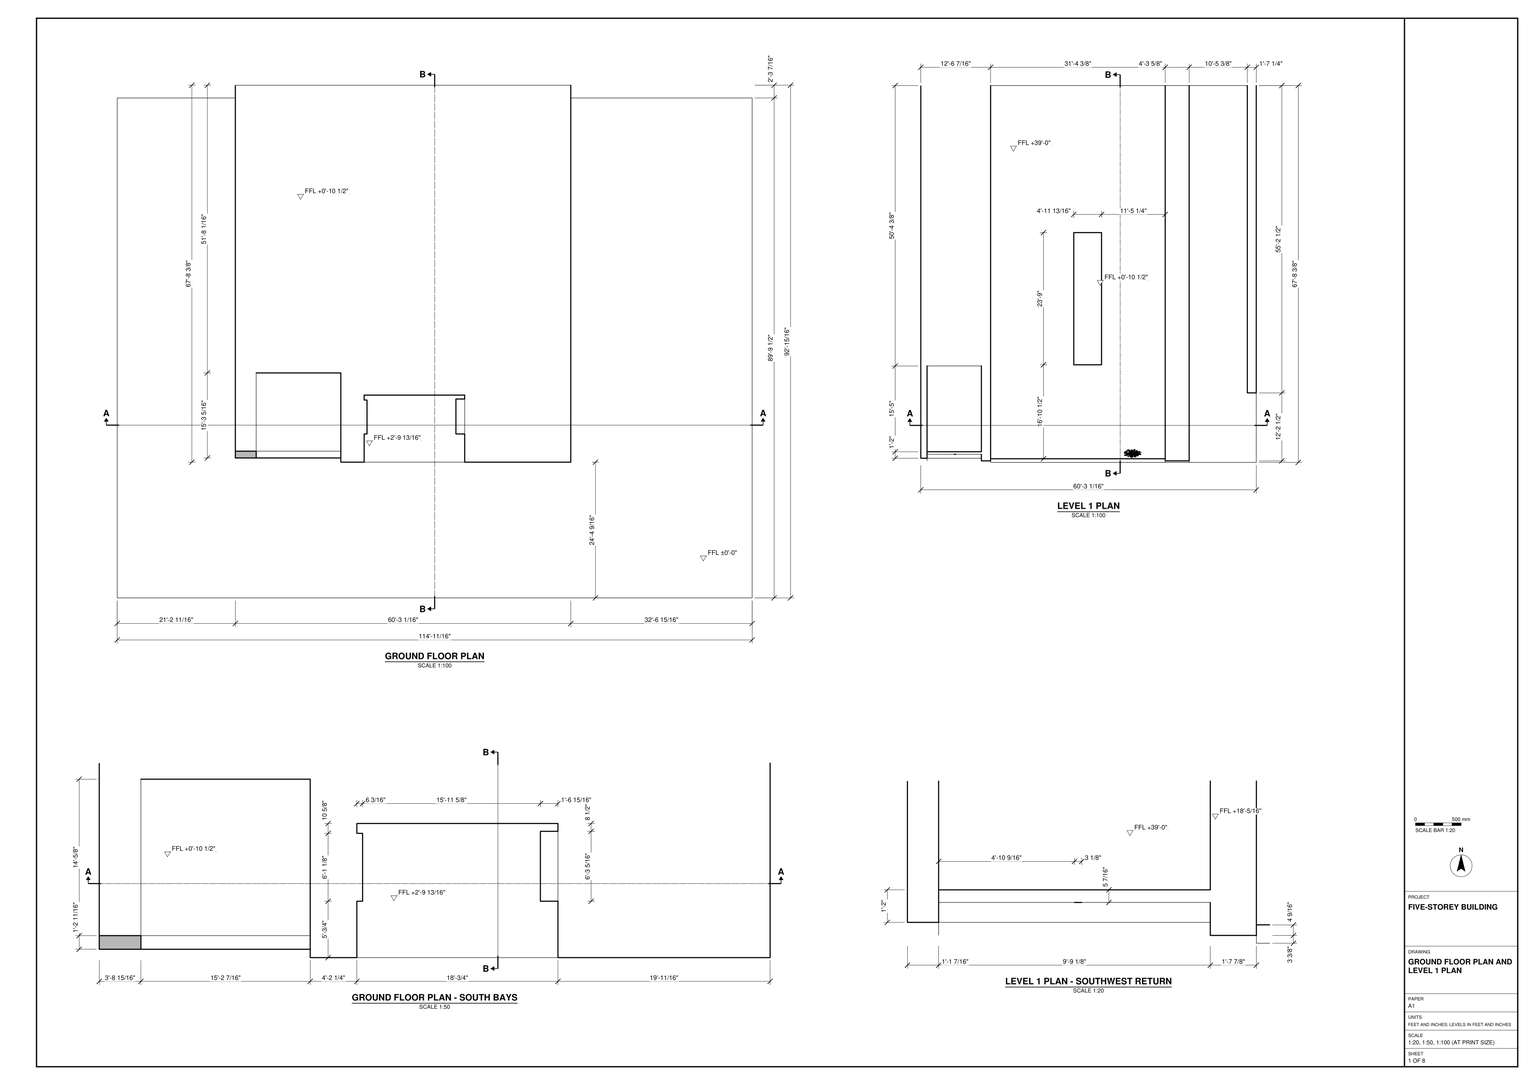
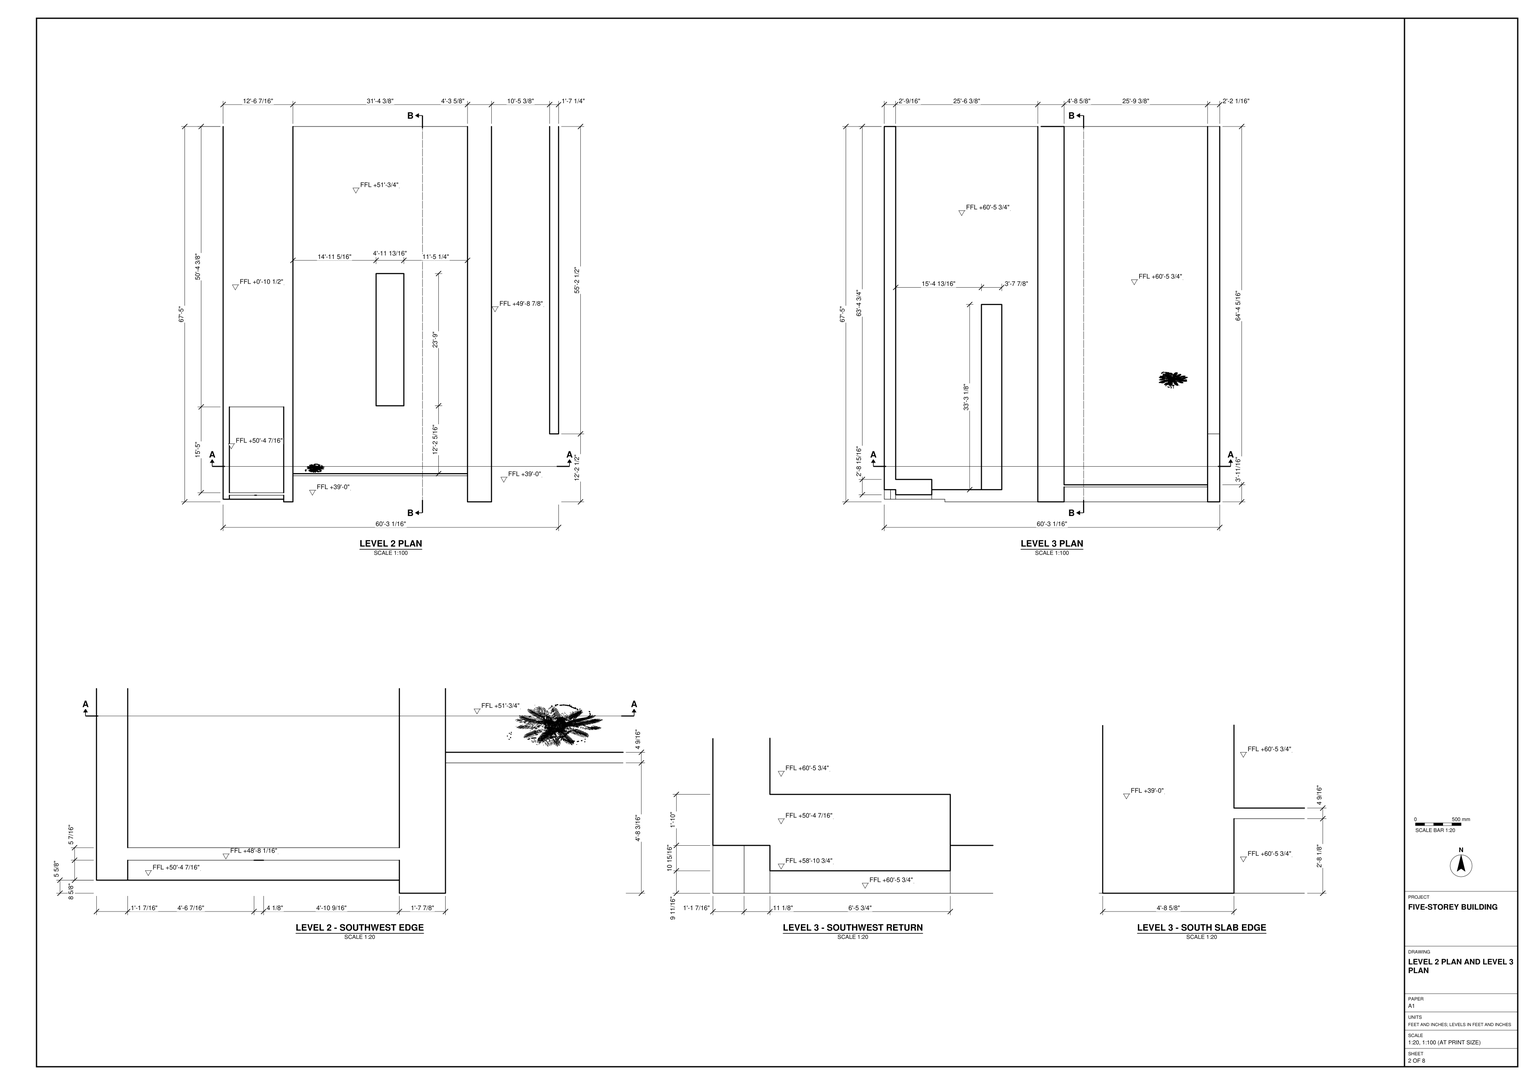
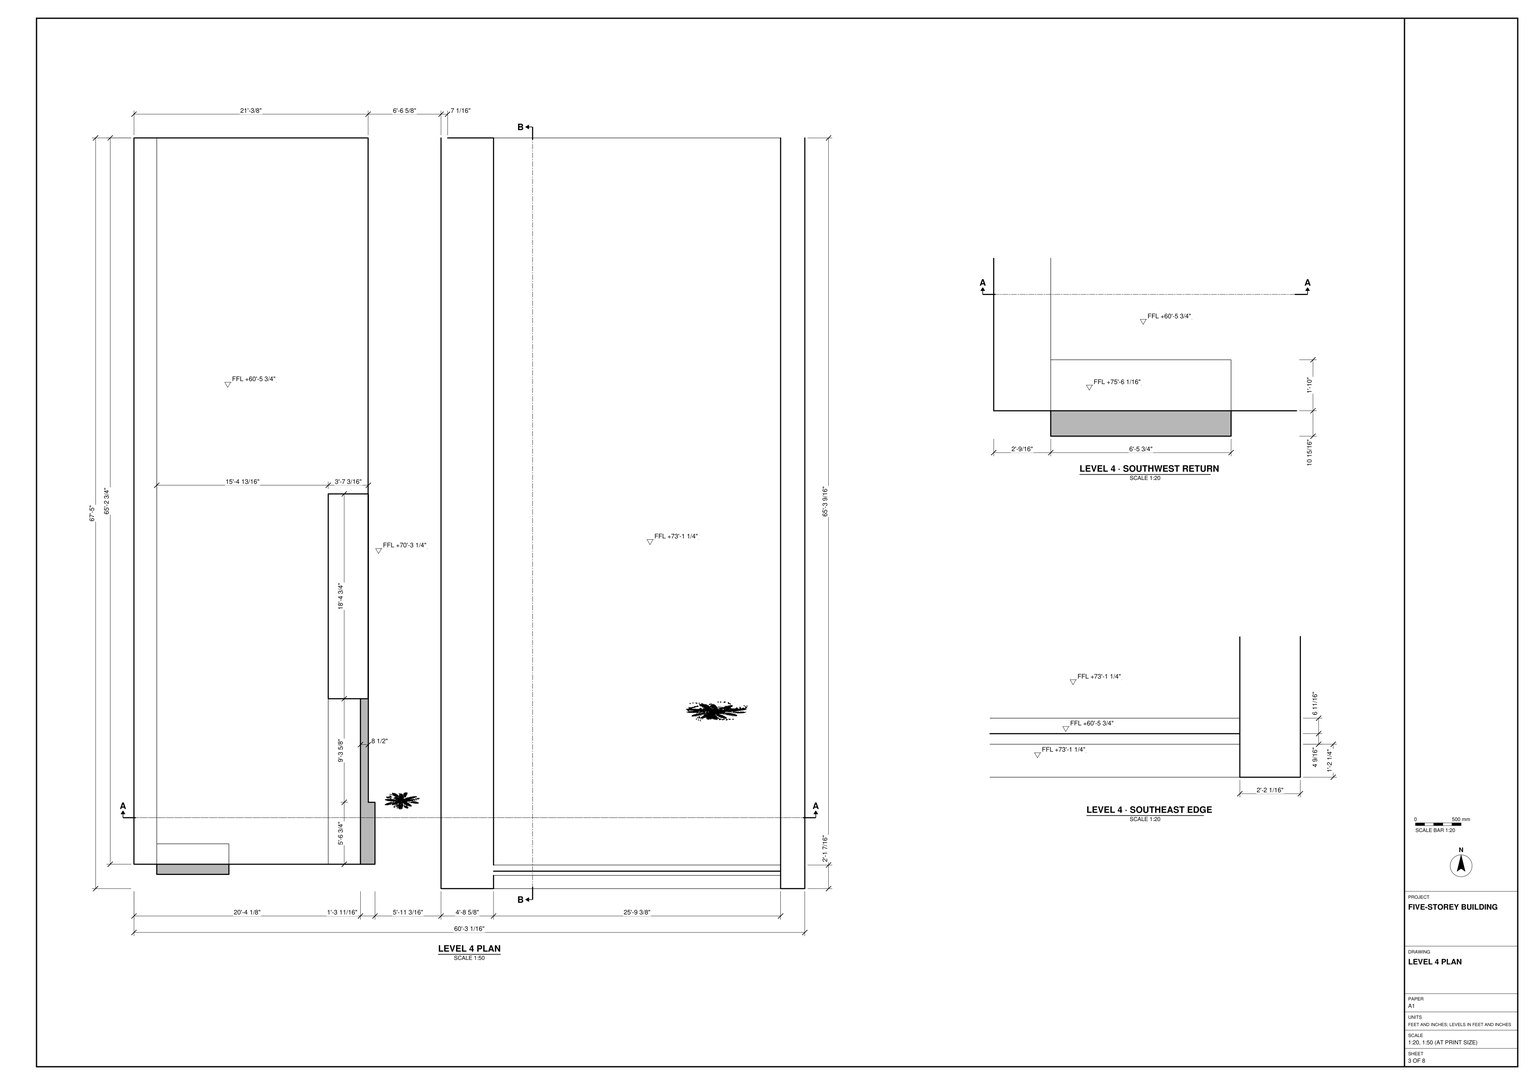
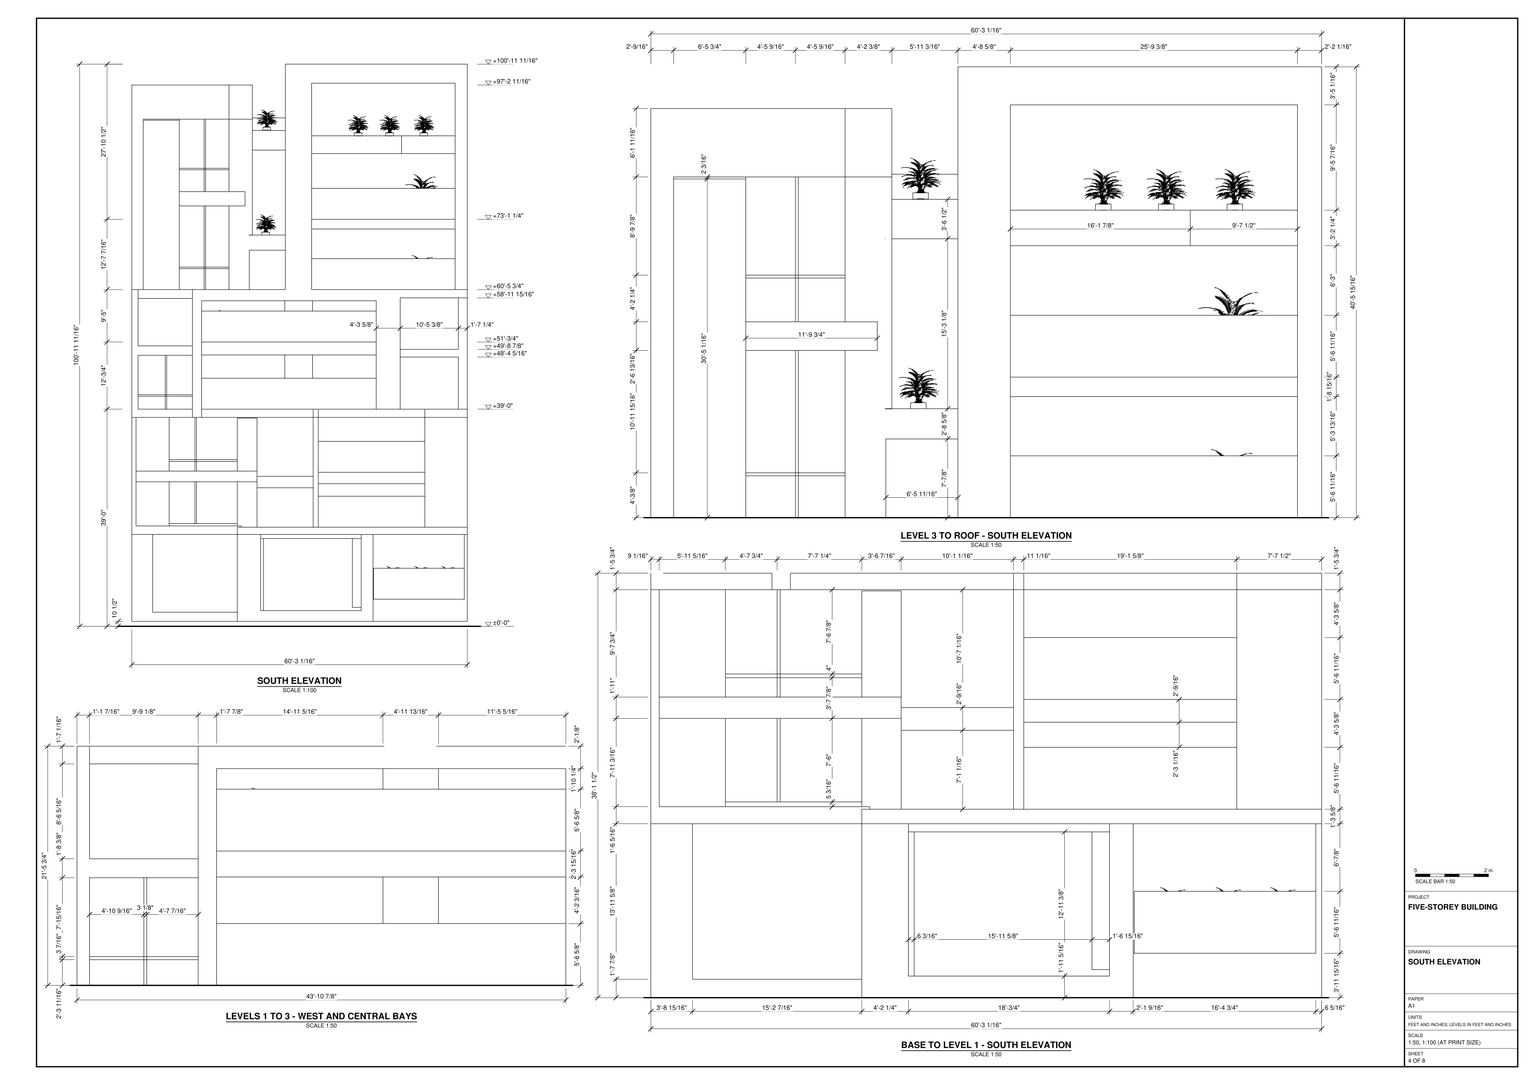
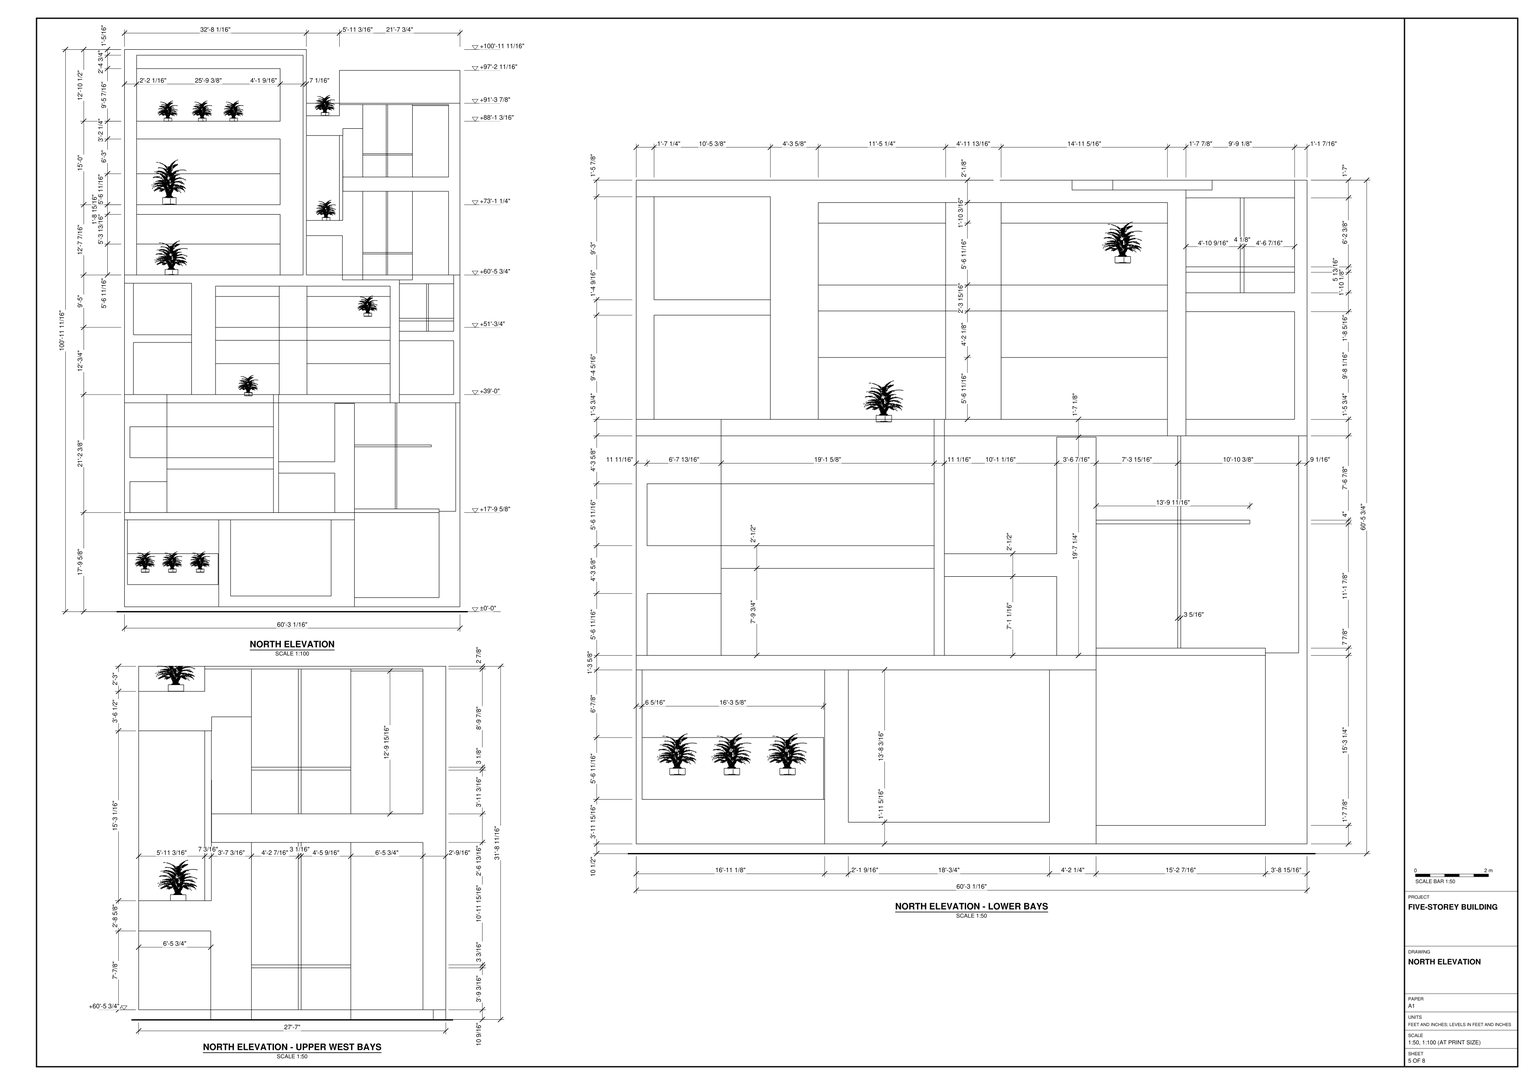
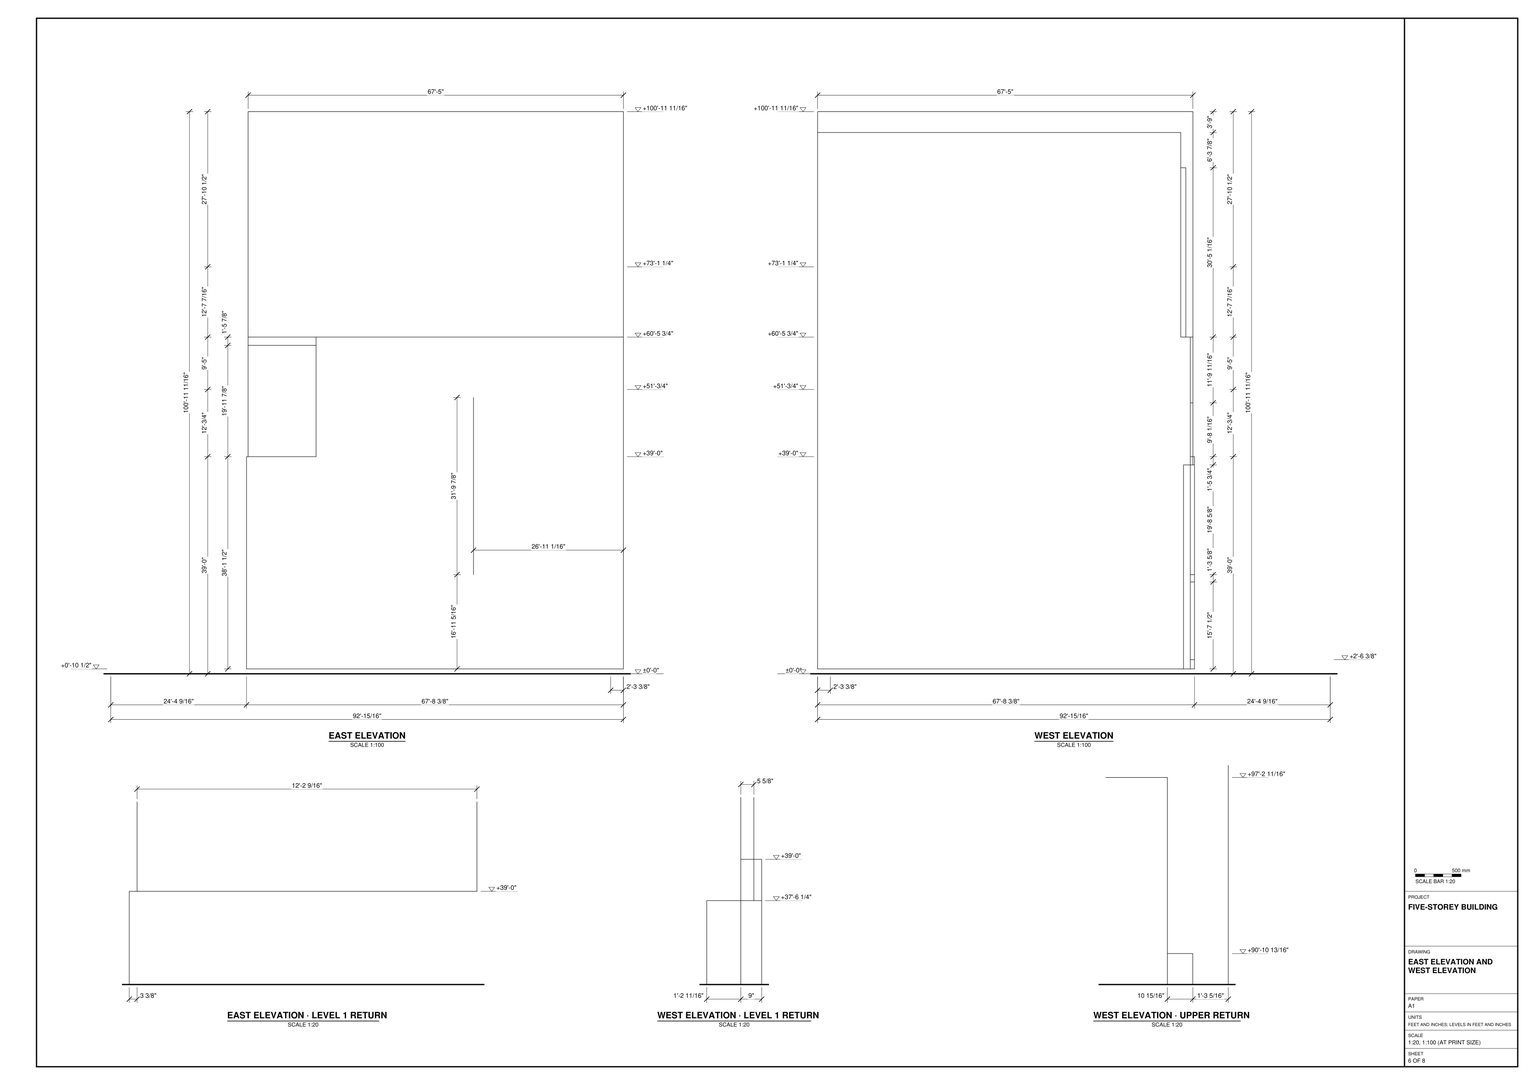
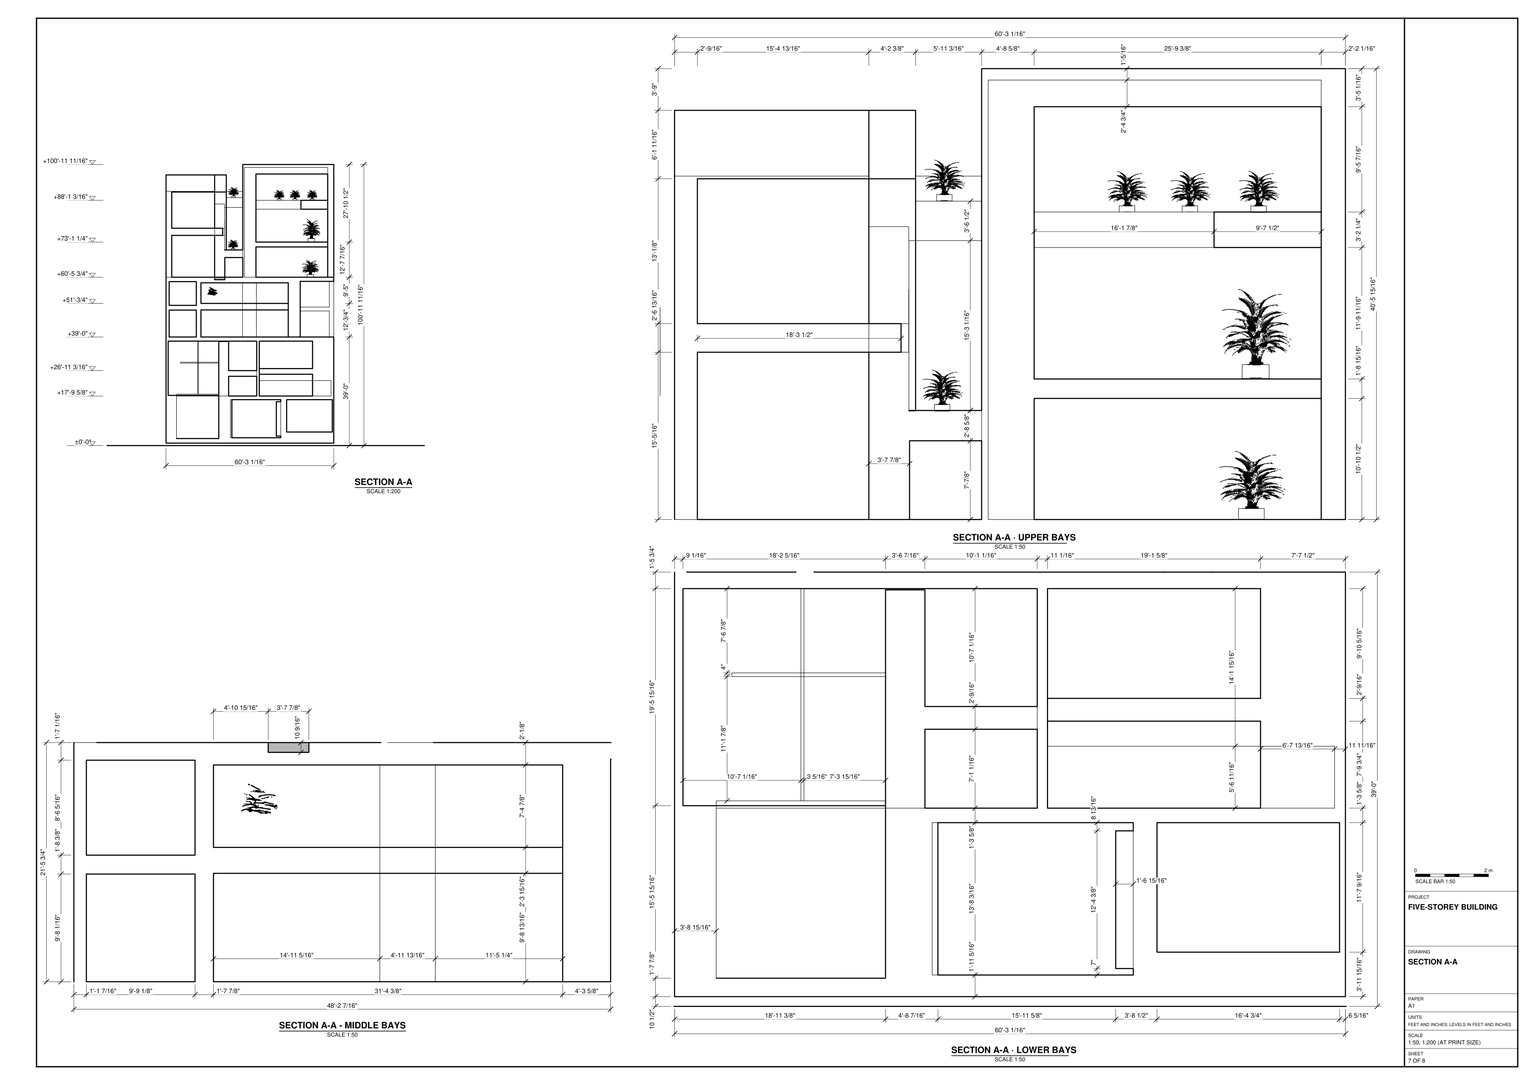
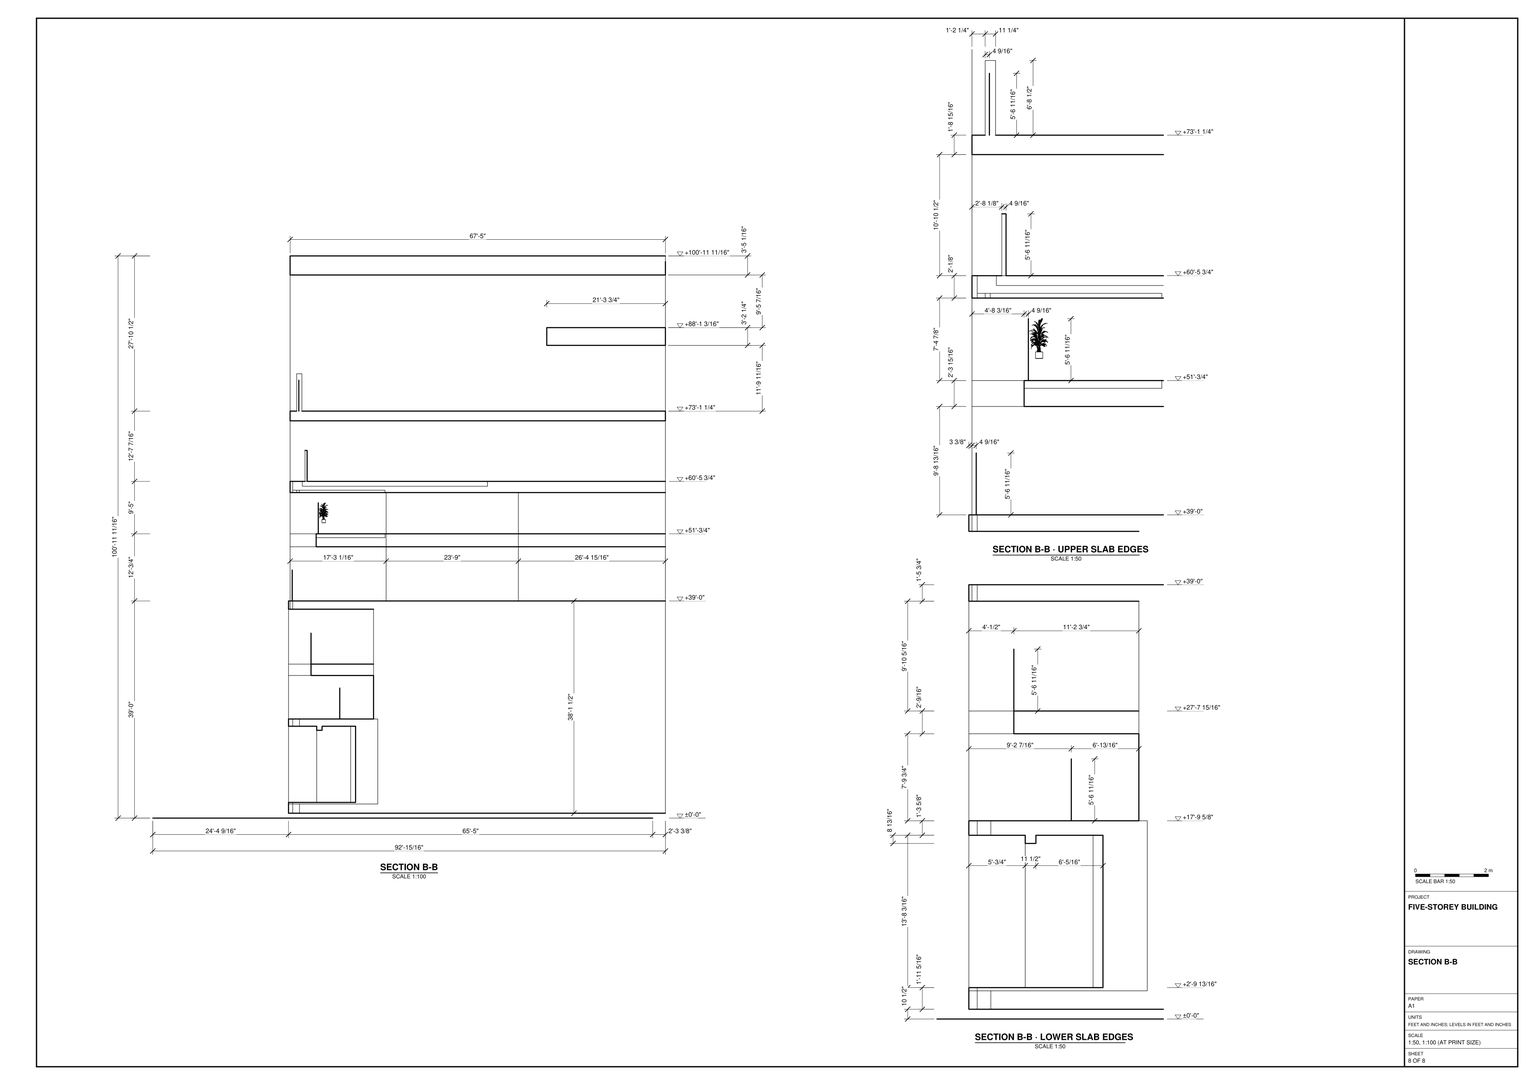
Build the five-storey building in SketchUp from task_files/diagram_01.pdf. Work in feet and inches. Including the site, the model shall span 114'-11/16" along X, 92'-15/16" along Y and 100'-11 11/16" along Z. Set the ground datum at ±0'-0" and the successive principal levels at +39'-0", +51'-3/4", +60'-5 3/4" and +73'-1 1/4".

Use the ground-floor plan to place the building on the site, leaving the open area to the south and the unequal margins to the west and east. Shape the south bays from the enlarged plan. Build each upper slab from its own outline rather than copying the ground footprint upwards. Preserve the long opening in the lower slabs, the stepped southwest returns and the change in height between the east and west portions at the top. Follow the sheets for wall thicknesses, openings, slab edges and roof profiles; include stairs, built-in joinery and main furniture where shown.

Keep walls, slabs and roof elements in separate groups or components, group each furniture or joinery piece separately, and use components for repeated parts. Plants and other loose or decorative items may be any suitable library components. Save one SketchUp model as output_files/five_storey_building_and_its_site.skp.

# SketchUp Ruby script. Lengths in inches.
U = 1.inch
M = Sketchup.active_model
def pt(a) = Geom::Point3d.new(a.map { |v| v * U })
def face(e, loops, mat)
  f = e.add_face(loops[0].map { |a| pt(a) })
  loops[1..].each { |l| e.add_face(l.map { |a| pt(a) }).erase! }
  f.material = f.back_material = mat if mat
  f
end
# faces: each face lists its corners as indices into pts; further lists are holes
def faces(e, pts, list, mat = nil) = list.each { |f| face(e, (f[0].is_a?(Array) ? f : [f]).map { |l| l.map { |i| pts[i] } }, mat) }
# xy, xz, yz: faces in a plane at the given z, y or x. An outline is a flat list of corners, or four numbers for a rectangle; further outlines are holes
def ring(l) = l.size == 4 ? [[l[0], l[1]], [l[2], l[1]], [l[2], l[3]], [l[0], l[3]]] : l.each_slice(2).to_a
def flat(e, list, mat, &to3) = list.each { |f| face(e, (f[0].is_a?(Array) ? f : [f]).map { |l| ring(l).map { |u, v| to3.(u, v) } }, mat) }
def xy(e, z, list, mat = nil) = flat(e, list, mat) { |x, y| [x, y, z] }
def xz(e, y, list, mat = nil) = flat(e, list, mat) { |x, z| [x, y, z] }
def yz(e, x, list, mat = nil) = flat(e, list, mat) { |y, z| [x, y, z] }
def lines(e, pts, list) = list.each { |a, b| e.add_line(pt(pts[a]), pt(pts[b])) }
# prism: a flat outline (further loops are holes) pulled along v
def prism(e, loops, v, mat = nil)
  f = face(e, loops, mat); d = Geom::Vector3d.new(v.map { |x| x * U })
  f.pushpull(f.normal.samedirection?(d) ? d.length : -d.length)
end
def box(e, o, s, mat = nil) = prism(e, [[o, [o[0] + s[0], o[1], o[2]], [o[0] + s[0], o[1] + s[1], o[2]], [o[0], o[1] + s[1], o[2]]]], [0, 0, s[2]], mat)
def at(x, y, z, deg = 0) = Geom::Transformation.translation(pt([x, y, z])) * Geom::Transformation.rotation(ORIGIN, Z_AXIS, deg.degrees)
def axes(o, x, y, z) = Geom::Transformation.new([*x, 0, *y, 0, *z, 0, *pt(o).to_a, 1])
def part(name) = M.definitions.add(name)
# library, detail: a bought-in or finely detailed component or shape, given as its bounding box
def library(name, o, s) = part(name).tap { |d| box(d.entities, o, s) }
def detail(e, o, s) = box(e.add_group.entities, o, s)
def put(e, d, t, mat = nil) = e.add_instance(d, t).tap { |i| i.material = mat if mat }
def group(e, t, mat = nil) = e.add_group.tap { |g| g.transformation = t; g.material = mat if mat }.entities
root = M.entities
M.materials.add("Niraj_Hair_Gray").color = [178, 178, 178]
M.materials.add("[Asphalt New]").color = [67, 60, 62]
M.materials.add("[Translucent Glass Gray]").color = [128, 128, 128]
M.materials["[Translucent Glass Gray]"].alpha = 0.5
c1 = library("plant_176_fbx.FBX\#1",[-22.43,-22.29,0],[44.86,44.58,89.56])
c2 = part("plant")
put(c2.entities,c1,axes([-237.41,482.42,160.98],[1.055,0,0],[0,0.5,0],[0,0,0.5]))
put(c2.entities,c1,axes([-237.41,591.17,160.98],[1.055,0,0],[0,0.5,0],[0,0,0.5]))
put(c2.entities,c1,axes([-237.41,699.92,160.98],[1.055,0,0],[0,0.5,0],[0,0,0.5]))
put(c2.entities,c1,axes([-237.41,808.67,160.98],[1.055,0,0],[0,0.5,0],[0,0,0.5]))
put(c2.entities,c1,axes([-237.41,917.42,160.98],[1.055,0,0],[0,0.5,0],[0,0,0.5]))
put(c2.entities,c1,axes([-237.41,1026.17,160.98],[1.055,0,0],[0,0.5,0],[0,0,0.5]))
put(c2.entities,c1,axes([-311.35,1134.92,160.98],[1.055,0,0],[0,0.5,0],[0,0,0.5]))
put(c2.entities,c1,axes([-379.16,1134.92,160.98],[1.055,0,0],[0,0.5,0],[0,0,0.5]))
put(c2.entities,c1,axes([-240.46,645.63,-18.48],[1.8357,0,0],[0,0.5,0],[0,0,1.09]))
put(c2.entities,c1,axes([-245.08,718.66,-169.93],[1.7513,0,0],[0,0.83,0],[0,0,0.83]))
put(c2.entities,c1,axes([-576.07,586.95,173.15],[1.055,0,0],[0,0.5,0],[0,0,0.5]))
put(c2.entities,c1,axes([-578.43,549.41,-53.08],[1.055,0,0],[0,0.5,0],[0,0,0.5]))
put(c2.entities,c1,axes([-410.75,470.8,-430.43],[1.055,0,0],[0,0.5,0],[0,0,0.5]))
put(c2.entities,c1,axes([-668.22,526.99,-259.24],[1.055,0,0],[0,0.5,0],[0,0,0.5]))
put(c2.entities,c1,axes([-246.96,495.71,-810.87],[1.055,0,0],[0,0.5,0],[0,0,0.5]))
put(c2.entities,c1,axes([-188.27,495.71,-810.87],[1.055,0,0],[0,0.5,0],[0,0,0.5]))
put(c2.entities,c1,axes([-306.89,495.71,-810.87],[1.055,0,0],[0,0.5,0],[0,0,0.5]))
xy(root,-10.52,[[0,0,1368.6875,1077.5]])
xy(root,0,[[482.05,292.54,977.74,292.54,977.74,1104.91,254.67,1104.91,254.67,316.23,482.05,316.23],[254.67,301.54,482.05,316.23]])
xy(root,19.86,[[299.59,301.54,482.05,316.23],[299.59,316.23,482.05,484.85]])
xy(root,23.3,[[532.33,292.54,749.08,292.54,749.08,437.1,532.33,437.1,532.33,426.45,538.51,426.45,538.51,353.31,532.33,353.31]])
xy(root,30.27,[[730.14,353.31,749.08,428.63]])
xy(root,47.93,[[774.63,292.54,971.41,430.29]])
xy(root,178.68,[[538.51,353.31,730.14,364.82],[730.14,364.82,749.08,428.63]])
xy(root,187.49,[[532.33,292.54,749.08,353.31],[774.63,292.54,971.41,430.29],[299.59,301.54,482.05,316.23],[538.51,364.82,538.51,426.45,532.33,426.45,532.33,437.1,749.08,437.1,749.08,364.82]])
xy(root,203.11,[[482.05,292.54,490.55,301.54],[490.55,292.54,524.51,341.2],[524.51,292.54,645.59,407.77],[656.63,292.54,886.23,402.95],[482.05,301.54,490.55,341.2],
  [656.63,402.95,886.23,475.79],[299.59,474.35,482.05,484.85]])
xy(root,205.8,[[263.76,301.54,490.55,301.54,490.55,341.2,482.05,341.2,482.05,445.35,299.59,445.35,299.59,407.77,263.76,407.77,263.76,364.84,335.07,364.84,335.07,354.66,263.76,354.66]])
xy(root,210.98,[[299.59,407.77,482.05,445.35],[299.59,445.35,482.05,474.35]])
xy(root,288.15,[[524.51,341.2,645.59,407.77]])
xy(root,296.88,[[656.63,341.04,886.23,475.79]])
xy(root,301.01,[[263.76,325.39,524.51,341.2]])
xy(root,312.68,[[524.51,341.2,645.59,407.77]])
xy(root,321.42,[[656.63,341.04,886.23,475.79]])
xy(root,324,[[263.76,325.39,524.51,341.2]])
xy(root,438.36,[[482.05,341.2,524.51,407.77]])
xy(root,439.72,[[405.13,292.54,405.13,295.91,385.26,295.91,385.26,301.54,263.76,301.54,263.76,354.66,335.07,354.66,335.07,364.84,263.76,364.84,263.76,407.77,645.59,407.77,645.59,292.54],[656.63,292.54,886.23,475.79]])
xy(root,457.5,[[405.13,292.54,781.5,300.48],[781.5,292.54,833.13,295.91],[833.13,292.54,977.74,292.54,977.74,442.44,958.52,442.44,958.52,1104.91,833.13,1104.91],[781.5,295.91,833.13,1104.91],[[405.13,300.48,781.5,1104.91],[584.42,502.95,644.24,787.95]],
  [268.13,301.54,385.26,310.14],[268.13,315.56,385.26,500.55]])
xy(root,569.81,[[833.13,442.44,958.52,1104.91]])
xy(root,573.5625,[[268.13,301.54,385.26,310.14],[268.13,310.14,385.26,315.56],[268.13,315.56,385.26,500.55]])
xy(root,574.32,[[405.13,352.1,781.5,1104.91]])
xy(root,586.375,[[833.13,442.44,958.52,1104.91]])
xy(root,593.9,[[268.13,301.54,385.26,310.14],[268.13,315.56,385.26,500.55]])
xy(root,602.26,[[405.13,352.1,781.5,356.66],[405.13,356.66,781.5,1104.91]])
xy(root,691.13,[[[405.13,295.91,781.5,1104.91],[584.42,502.95,644.24,787.95]]])
xy(root,696.24,[[268.13,301.54,385.26,310.14],[268.13,310.14,385.26,315.56],[268.13,315.56,385.26,500.55]])
xy(root,697.4,[[833.13,295.91,833.13,1104.91,958.52,1104.91,958.52,442.44,977.74,442.44,977.74,295.91]])
xy(root,704.68,[[464.09,322.17,507.95,721.28]])
xy(root,715.25,[[385.26,295.91,585.65,295.91,585.65,1104.91,279.26,1104.91,279.26,344.16,357.01,344.16,357.01,301.54,385.26,301.54],[642.25,295.91,951.65,328.06],[951.65,295.91,977.74,442.44],[254.67,301.54,268.13,322.17],[268.13,301.54,279.26,322.17],
  [279.26,301.54,357.01,311.23],[642.25,332.62,951.65,1104.91],[951.65,442.44,977.74,1104.91]])
xy(root,781.9375,[[642.25,328.06,951.65,332.62]])
xy(root,800.12,[[507.95,322.17,585.65,721.28]])
xy(root,832.47,[[507.29,322.17,514.45,388.92]])
xy(root,832.75,[[507.29,322.17,585.65,721.28]])
xy(root,845.76,[[642.25,295.91,951.65,1104.91]])
xy(root,866.7,[[642.25,295.91,951.65,310.14],[642.25,321.36,951.65,1104.91]])
xy(root,895.54,[[279.26,322.17,357.01,344.16],[357.01,322.17,357.01,344.16,279.26,344.16,279.26,1104.91,507.04,1104.91,507.04,500.55,464.09,500.55,464.09,322.17],[464.09,322.17,498.78,500.55]])
xy(root,916.6,[[507.04,500.55,507.29,721.28]])
xy(root,926.35,[[279.26,322.17,464.09,322.17,464.09,500.55,507.04,500.55,507.04,1104.91,279.26,1104.91],[464.09,322.17,498.78,500.55]])
xy(root,962.91,[[507.04,500.55,507.29,721.28]])
xy(root,1008.41,[[836.15,295.91,951.65,849.18],[642.25,849.18,951.65,1104.91]])
xy(root,1015.83,[[507.29,388.92,585.65,721.28],[507.04,510.8125,507.29,721.28]])
xy(root,1030.89,[[507.04,510.8125,498.78,721.28,507.04,721.28]])
xy(root,1046.68,[[836.15,295.91,951.65,849.18],[642.25,849.18,951.65,1104.91]])
xy(root,1058.33,[[514.45,388.92,585.65,721.28]])
xy(root,1080.29,[[279.26,311.23,357.01,322.17]])
xy(root,1082.48,[[279.26,322.17,514.45,1104.91]])
xy(root,1156.1875,[[254.67,322.17,464.09,322.17,464.09,721.28,514.45,721.28,514.45,1104.91,254.67,1104.91],[464.09,322.17,514.45,721.28]])
xy(root,1160.125,[[642.25,295.91,951.65,1104.91]])
xy(root,1201.1875,[[585.65,295.91,977.74,1104.91]])
xz(root,292.54,[[482.05,0,774.63,0,774.63,187.49,749.08,187.49,749.08,23.3,532.33,23.3,532.33,187.49,482.05,187.49],[774.63,0,977.74,0,977.74,187.49,971.41,187.49,971.41,47.93,774.63,47.93],[482.05,187.49,977.74,203.11],[645.59,203.11,656.63,439.72],[886.23,203.11,977.74,439.72],
  [405.13,439.72,645.59,457.5],[645.59,439.72,656.63,457.5],[656.63,439.72,886.23,457.5],[886.23,439.72,977.74,457.5]])
xz(root,295.91,[[385.26,439.72,405.13,439.72,405.13,691.13,781.5,691.13,781.5,457.5,833.13,457.5,833.13,697.4,977.74,697.4,977.74,715.25,642.25,715.25,642.25,1160.125,951.65,1160.125,951.65,715.25,977.74,715.25,977.74,1201.1875,585.65,1201.1875,585.65,715.25,385.26,715.25],[642.25,845.76,951.65,866.7],[836.15,1008.41,951.65,1046.68]])
xz(root,300.48,[[405.13,457.5,781.5,524.1875]])
xz(root,301.54,[[299.59,19.86,482.05,187.49],[254.67,187.49,482.05,187.49,482.05,203.11,490.55,203.11,490.55,205.8,263.76,205.8,263.76,439.72,254.67,439.72],[254.67,439.72,385.26,439.72,385.26,457.5,268.13,457.5,268.13,573.5625,385.26,573.5625,385.26,593.9,268.13,593.9,268.13,715.25,254.67,715.25],[268.13,696.24,385.26,715.25]])
xz(root,301.54,[[254.67,0,482.05,0,482.05,19.86,299.59,19.86,299.59,187.49,254.67,187.49]],"Niraj_Hair_Gray")
xz(root,301.54,[[268.13,593.9,385.26,696.24]],"[Translucent Glass Gray]")
xz(root,310.14,[[326.7,457.5,329.83,485.15],[268.13,485.15,326.7,488.57],[326.7,485.15,329.83,488.57],[329.83,485.15,385.26,488.57],[326.7,488.57,329.83,573.5625],
  [322.59,593.9,326.7,616.03],[268.13,616.03,322.59,621.87],[322.59,616.03,326.7,621.87],[326.7,616.03,385.26,621.87],[322.59,621.87,326.7,696.24]],"[Asphalt New]")
xz(root,311.23,[[279.26,715.25,357.01,1080.29]])
xz(root,314.7,[[642.25,866.7,951.65,933.39]])
xz(root,315.56,[[268.13,457.5,385.26,573.5625]],"[Translucent Glass Gray]")
xz(root,316.23,[[254.67,0,254.67,439.72,263.76,439.72,263.76,205.8,490.55,205.8,490.55,203.11,482.05,203.11,482.05,187.49,299.59,187.49,299.59,19.86,482.05,19.86,482.05,0]])
xz(root,322.17,[[464.09,704.68,507.95,704.68,507.95,800.12,585.65,800.12,585.65,832.75,514.45,832.75,514.45,832.47,507.29,832.47,507.29,832.75,514.45,832.75,514.45,1082.48,464.09,1082.48,464.09,926.35,498.78,926.35,498.78,895.54,464.09,895.54],[254.67,715.25,279.26,715.25,279.26,1082.48,464.09,1082.48,464.09,1156.1875,254.67,1156.1875],[507.29,832.47,514.45,832.75],[279.26,895.54,357.01,926.35],[357.01,895.54,498.78,926.35],
  [279.26,926.35,357.01,1080.29],[279.26,1080.29,357.01,1082.48],[464.09,1082.48,514.45,1156.1875]])
xz(root,322.17,[[410.55,715.25,413.64,760.41],[357.01,760.41,410.55,763.61],[410.55,760.41,413.64,763.61],[413.64,760.41,464.09,763.61],[410.55,763.61,413.64,895.54],
  [410.55,926.35,413.58,973.52],[357.01,973.52,410.55,976.625],[410.55,973.52,413.58,976.625],[413.58,973.52,464.09,976.625],[410.55,976.625,413.58,1082.48]],"[Asphalt New]")
xz(root,322.17,[[357.01,704.68,464.09,704.68,464.09,760.41,413.64,760.41,413.64,715.25,410.55,715.25,410.55,760.41,357.01,760.41],[357.01,763.61,410.55,895.54],[413.64,763.61,464.09,895.54],[357.01,926.35,410.55,973.52],[413.58,926.35,464.09,973.52],
  [357.01,976.625,410.55,1082.48],[413.58,976.625,464.09,1082.48]],"[Translucent Glass Gray]")
xz(root,325.39,[[775.78,47.93,971.41,114.62],[263.76,301.01,524.51,324]])
xz(root,332.62,[[642.25,715.25,951.65,781.9375]])
xz(root,341.04,[[656.63,296.88,886.23,321.42],[656.63,321.42,966.02,388.1]])
xz(root,341.2,[[482.05,203.11,490.55,205.8],[490.55,203.11,524.51,203.11,524.51,301.01,482.05,301.01,482.05,205.8,490.55,205.8],[524.51,288.15,645.59,312.68],[263.76,301.01,482.05,324],[482.05,301.01,524.51,324],
  [482.05,324,524.51,438.36]])
xz(root,344.16,[[279.26,715.25,357.01,895.54]])
xz(root,352.1,[[405.13,574.32,781.5,602.26]])
xz(root,353.31,[[532.33,23.3,538.51,178.68],[730.14,30.27,749.08,178.68],[532.33,178.68,749.08,187.49]])
xz(root,354.66,[[263.76,205.8,335.07,439.72]])
xz(root,356.66,[[405.13,602.26,781.5,668.94]])
xz(root,364.82,[[538.51,178.68,749.08,187.49]])
xz(root,364.84,[[263.76,205.8,335.07,439.72]])
xz(root,388.92,[[507.29,832.47,514.45,1015.83],[514.45,1015.83,585.65,1058.33]])
xz(root,402.95,[[656.63,203.11,966.02,269.8]])
xz(root,407.77,[[482.05,203.11,482.05,438.36,524.51,438.36,524.51,312.68,645.59,312.68,645.59,288.15,524.51,288.15,524.51,203.11]])
xz(root,407.77,[[390.82,210.98,394.125,344.87],[316.36,344.87,390.82,348.87],[390.82,344.87,394.125,348.87],[394.125,344.87,482.05,348.87],[390.82,348.87,394.125,439.72]],"[Asphalt New]")
xz(root,407.77,[[524.51,203.11,645.59,288.15],[263.76,205.8,299.59,205.8,299.59,210.98,390.82,210.98,390.82,344.87,316.36,344.87,316.36,348.87,390.82,348.87,390.82,439.72,263.76,439.72],[394.125,210.98,482.05,344.87],[524.51,312.68,645.59,312.68,645.59,439.72,394.125,439.72,394.125,348.87,482.05,348.87,482.05,438.36,524.51,438.36]],"[Translucent Glass Gray]")
xz(root,426.45,[[532.33,23.3,538.51,187.49]])
xz(root,428.63,[[730.14,30.27,749.08,178.68]])
xz(root,437.1,[[532.33,23.3,749.08,187.49]])
xz(root,442.44,[[958.52,457.5,977.74,457.5,977.74,697.4,958.52,697.4,958.52,586.375,833.13,586.375,833.13,569.81,958.52,569.81]])
xz(root,445.35,[[299.59,205.8,482.05,210.98]])
xz(root,474.35,[[299.59,203.11,482.05,210.98]])
xz(root,475.79,[[656.63,203.11,886.23,296.88]],"[Translucent Glass Gray]")
xz(root,484.85,[[299.59,19.86,482.05,203.11]])
xz(root,500.55,[[464.09,895.54,498.78,926.35],[498.78,895.54,507.04,926.35],[507.04,916.6,507.29,962.91]])
xz(root,502.95,[[584.42,457.5,644.24,691.13]])
xz(root,721.28,[[464.09,704.68,464.09,1030.89,507.04,1030.89,507.04,1015.83,507.29,1015.83,507.29,962.91,507.04,962.91,507.04,916.6,507.29,916.6,507.29,832.75,585.65,832.75,585.65,800.12,507.95,800.12,507.95,704.68],[507.04,1015.83,507.04,1030.89,464.09,1030.89,464.09,1156.1875,514.45,1156.1875,514.45,1058.33,585.65,1058.33,585.65,1015.83]])
xz(root,787.95,[[584.42,457.5,644.24,691.13]])
xz(root,849.18,[[642.25,1008.41,836.15,1046.68]])
xz(root,1104.91,[[254.67,715.25,254.67,1085.35,514.45,1085.35,514.45,1082.48,279.26,1082.48,279.26,926.35,507.04,926.35,507.04,895.54,279.26,895.54,279.26,715.25],[592.71,715.25,592.71,1188.875,951.65,1188.875,951.65,1160.125,642.25,1160.125,642.25,1046.68,951.65,1046.68,951.65,1008.41,642.25,1008.41,642.25,866.7,951.65,866.7,951.65,845.76,642.25,845.76,642.25,715.25],[254.67,1085.35,514.45,1156.1875]])
yz(root,254.67,[[301.54,0,316.23,439.72],[316.23,0,1104.91,0,1104.91,1156.1875,322.17,1156.1875,322.17,715.25,301.54,715.25,301.54,439.72,316.23,439.72]])
yz(root,263.76,[[301.54,205.8,316.23,439.72],[[316.23,205.8,354.66,439.72],[325.39,301.01,341.2,324]],[364.84,205.8,407.77,439.72]])
yz(root,268.13,[[301.54,457.5,310.14,573.5625],[310.14,457.5,315.56,573.5625],[315.56,457.5,500.55,573.5625],[301.54,593.9,310.14,696.24],[315.56,593.9,500.55,696.24]])
yz(root,279.26,[[311.23,715.25,322.17,1080.29],[344.16,715.25,1104.91,895.54],[322.17,926.35,1104.91,1082.48]])
yz(root,299.59,[[301.54,19.86,316.23,187.49],[407.77,205.8,445.35,210.98]])
yz(root,335.07,[[354.66,205.8,364.84,439.72]])
yz(root,357.01,[[311.23,715.25,322.17,1080.29],[322.17,715.25,344.16,895.54]])
yz(root,385.26,[[295.91,439.72,301.54,457.5],[295.91,457.5,310.14,573.5625],[315.56,457.5,500.55,573.5625],[295.91,573.5625,301.54,715.25],[301.54,593.9,310.14,696.24],
  [315.56,593.9,500.55,696.24]])
yz(root,405.13,[[292.54,439.72,295.91,457.5],[295.91,457.5,1104.91,574.32],[295.91,574.32,352.1,602.26],[295.91,602.26,1104.91,691.13]])
yz(root,464.09,[[322.17,704.68,322.17,895.54,500.55,895.54,500.55,926.35,322.17,926.35,322.17,1156.1875,721.28,1156.1875,721.28,704.68]])
yz(root,482.05,[[292.54,0,301.54,19.86],[292.54,19.86,301.54,187.49],[301.54,19.86,301.54,187.49,316.23,187.49,316.23,203.11,341.2,203.11,341.2,205.8,407.77,205.8,407.77,203.11,484.85,203.11,484.85,19.86],[292.54,187.49,301.54,203.11],[301.54,187.49,316.23,203.11],
  [407.77,203.11,474.35,203.11,474.35,210.98,445.35,210.98,445.35,205.8,407.77,205.8],[341.2,205.8,407.77,438.36],[407.77,205.8,445.35,210.98]])
yz(root,490.55,[[301.54,203.11,341.2,205.8]])
yz(root,498.78,[[322.17,895.54,500.55,926.35]])
yz(root,507.04,[[500.55,895.54,721.28,916.6],[721.28,895.54,1104.91,926.35],[500.55,916.6,721.28,926.35],[500.55,926.35,721.28,962.91],[510.8125,1015.83,721.28,1030.89]])
yz(root,507.29,[[322.17,832.47,388.92,832.75],[388.92,832.75,721.28,832.75,721.28,916.6,500.55,916.6,500.55,962.91,388.92,962.91],[388.92,962.91,721.28,1015.83]])
yz(root,507.95,[[322.17,704.68,721.28,800.12]])
yz(root,514.45,[[322.17,832.47,388.92,1058.33],[322.17,1058.33,721.28,1082.48],[322.17,1082.48,721.28,1156.1875],[721.28,1082.48,1104.91,1156.1875]])
yz(root,524.51,[[341.2,203.11,407.77,288.15],[325.39,301.01,341.2,324],[341.2,312.68,407.77,438.36]])
yz(root,532.33,[[292.54,23.3,353.31,187.49],[426.45,23.3,437.1,187.49]])
yz(root,538.51,[[353.31,23.3,426.45,23.3,426.45,187.49,364.82,187.49,364.82,178.68,353.31,178.68]])
yz(root,584.42,[[502.95,457.5,787.95,691.13]])
yz(root,585.65,[[[295.91,715.25,1104.91,1201.1875],[388.92,1015.83,721.28,1058.33],[322.17,800.12,721.28,832.75]]])
yz(root,642.25,[[295.91,715.25,328.06,715.25,328.06,781.9375,332.62,781.9375,332.62,715.25,1104.91,715.25,1104.91,845.76,295.91,845.76],[295.91,866.7,310.14,866.7,310.14,947.2,321.36,947.2,321.36,866.7,1104.91,866.7,1104.91,1008.41,849.18,1008.41,849.18,1046.68,1104.91,1046.68,1104.91,1160.125,295.91,1160.125]])
yz(root,644.24,[[502.95,457.5,787.95,691.13]])
yz(root,645.59,[[292.54,203.11,292.54,439.72,407.77,439.72,407.77,312.68,341.2,312.68,341.2,288.15,407.77,288.15,407.77,203.11]])
yz(root,656.63,[[292.54,203.11,475.79,296.88],[292.54,296.88,341.04,321.42],[341.04,296.88,475.79,321.42],[292.54,321.42,475.79,439.72]])
yz(root,730.14,[[353.31,30.27,428.63,178.68]])
yz(root,749.08,[[292.54,23.3,292.54,187.49,353.31,187.49,353.31,30.27,428.63,30.27,428.63,178.68,364.82,178.68,364.82,187.49,437.1,187.49,437.1,23.3]])
yz(root,774.63,[[292.54,47.93,430.29,187.49]])
yz(root,781.5,[[295.91,457.5,1104.91,574.32],[295.91,574.32,352.1,602.26],[352.1,574.32,1104.91,602.26],[295.91,602.26,1104.91,691.13]])
yz(root,833.13,[[295.91,457.5,1104.91,457.5,1104.91,569.81,442.44,569.81,442.44,586.375,1104.91,586.375,1104.91,697.4,295.91,697.4]])
yz(root,836.15,[[295.91,1008.41,849.18,1046.68]])
yz(root,886.23,[[292.54,203.11,475.79,296.88],[292.54,296.88,341.04,321.42],[292.54,321.42,475.79,439.72]])
yz(root,951.65,[[295.91,715.25,295.91,845.76,1104.91,845.76,1104.91,715.25,332.62,715.25,332.62,781.9375,328.06,781.9375,328.06,715.25],[328.06,715.25,332.62,781.9375],[295.91,845.76,1104.91,845.76,1104.91,866.7,321.36,866.7,321.36,947.2,310.14,947.2,310.14,866.7,295.91,866.7],[295.91,866.7,295.91,1008.41,1104.91,1008.41,1104.91,866.7,321.36,866.7,321.36,947.2,310.14,947.2,310.14,866.7],[295.91,1008.41,1104.91,1046.68],
  [295.91,1046.68,1104.91,1160.125]])
yz(root,958.52,[[442.44,457.5,1104.91,569.81],[442.44,586.375,1104.91,697.4]])
yz(root,971.41,[[292.54,47.93,430.29,187.49]])
yz(root,977.74,[[292.54,0,1104.91,0,1104.91,715.25,442.44,715.25,442.44,457.5,292.54,457.5],[295.91,697.4,442.44,715.25],[295.91,715.25,1104.91,1201.1875]])
p = [[507.04,322.17,1015.83],[507.29,322.17,1015.83],[507.29,388.92,962.91],[507.29,322.17,962.91],[585.65,1104.91,1085.35],[514.45,1104.91,1085.35],
  [268.13,301.54,457.5],[268.13,295.91,457.5],[2384.64,781.82,585.17],[2384.64,781.82,203.3]]
lines(root,p,[[0,1],[2,3],[4,5],[6,7],[8,9]])
put(root,c2,at(1121.6,-159.18,885.18))
